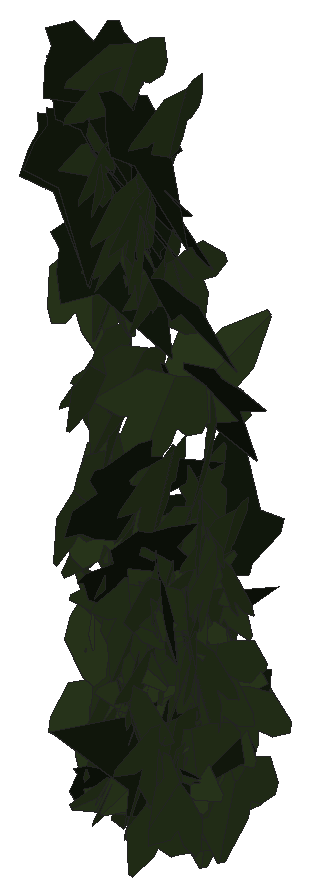
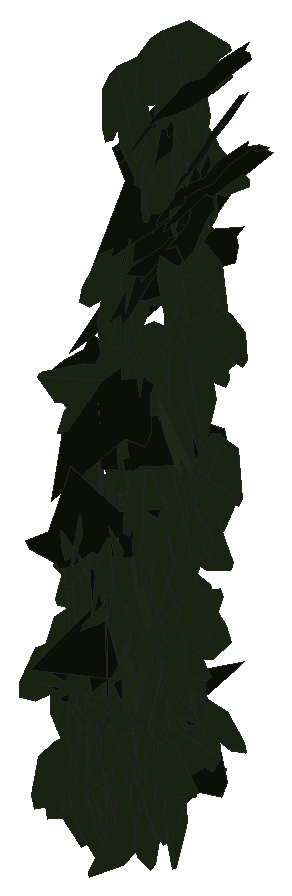
# SketchUp Ruby script. Lengths in inches.
U = 1.inch
M = Sketchup.active_model
def pt(a) = Geom::Point3d.new(a.map { |v| v * U })
def face(e, loops, mat)
  f = e.add_face(loops[0].map { |a| pt(a) })
  loops[1..].each { |l| e.add_face(l.map { |a| pt(a) }).erase! }
  f.material = f.back_material = mat if mat
  f
end
# faces: each face lists its corners as indices into pts; further lists are holes
def faces(e, pts, list, mat = nil) = list.each { |f| face(e, (f[0].is_a?(Array) ? f : [f]).map { |l| l.map { |i| pts[i] } }, mat) }
# xy, xz, yz: faces in a plane at the given z, y or x. An outline is a flat list of corners, or four numbers for a rectangle; further outlines are holes
def ring(l) = l.size == 4 ? [[l[0], l[1]], [l[2], l[1]], [l[2], l[3]], [l[0], l[3]]] : l.each_slice(2).to_a
def flat(e, list, mat, &to3) = list.each { |f| face(e, (f[0].is_a?(Array) ? f : [f]).map { |l| ring(l).map { |u, v| to3.(u, v) } }, mat) }
def xy(e, z, list, mat = nil) = flat(e, list, mat) { |x, y| [x, y, z] }
def xz(e, y, list, mat = nil) = flat(e, list, mat) { |x, z| [x, y, z] }
def yz(e, x, list, mat = nil) = flat(e, list, mat) { |y, z| [x, y, z] }
def lines(e, pts, list) = list.each { |a, b| e.add_line(pt(pts[a]), pt(pts[b])) }
# prism: a flat outline (further loops are holes) pulled along v
def prism(e, loops, v, mat = nil)
  f = face(e, loops, mat); d = Geom::Vector3d.new(v.map { |x| x * U })
  f.pushpull(f.normal.samedirection?(d) ? d.length : -d.length)
end
def box(e, o, s, mat = nil) = prism(e, [[o, [o[0] + s[0], o[1], o[2]], [o[0] + s[0], o[1] + s[1], o[2]], [o[0], o[1] + s[1], o[2]]]], [0, 0, s[2]], mat)
def at(x, y, z, deg = 0) = Geom::Transformation.translation(pt([x, y, z])) * Geom::Transformation.rotation(ORIGIN, Z_AXIS, deg.degrees)
def axes(o, x, y, z) = Geom::Transformation.new([*x, 0, *y, 0, *z, 0, *pt(o).to_a, 1])
def part(name) = M.definitions.add(name)
# library, detail: a bought-in or finely detailed component or shape, given as its bounding box
def library(name, o, s) = part(name).tap { |d| box(d.entities, o, s) }
def detail(e, o, s) = box(e.add_group.entities, o, s)
def put(e, d, t, mat = nil) = e.add_instance(d, t).tap { |i| i.material = mat if mat }
def group(e, t, mat = nil) = e.add_group.tap { |g| g.transformation = t; g.material = mat if mat }.entities
root = M.entities
M.materials.add("efeu1").color = [18, 25, 13]
M.materials.add("efeu2").color = [43, 57, 29]
c1 = part("ivyleaf_10")
p = [[0,0.5,-0.03],[-0.0625,2.02,-0.43],[-0.19,2.01,-0.46],[-0.54,1.05,-0.29],[-0.52,0.625,-0.18],[-0.83,0.76,-0.28],
  [-1.16,0.64,-0.33],[-1.15,0.33,-0.24],[-0.77,-0.39,0.02],[-0.3,-0.51,0.16],[0.04,-0.48,0.23],[-0.02,2.01,-0.4375],
  [-0.06,2.01,-0.43],[0.04,-0.49,0.23],[0.67,-0.49,0.14],[1.38,0.36,-0.2],[1.375,0.51,-0.24],[0.81,0.65,-0.19],
  [0.62,0.59,-0.15],[0.6,1.09,-0.28],[0.5,1.23,-0.31]]
faces(c1.entities,p,[[0,1,2,3,4,5,6,7,8,9,10],[11,12,0,13,14,15,16,17,18,19,20]],"efeu2")
c2 = part("ivyleaf_9")
p = [[1.54,2.16,1.25],[1.36,2.04,1.19],[-0.21,0.99,0.68],[-0.71,1.11,0.82],[-0.85,0.86,0.67],[-0.8,0.17,0.21],
  [-0.9,-0.01,0.1],[-0.67,-0.16,-0.02],[-0.08,-0.08,-0.05],[-0.03,-0.6,-0.4],[0.65,-0.88,-0.66],[0.83,-0.6,-0.49],
  [1.29,-0.42,-0.43],[1.8125,-0.07,-0.26],[1.21,0.44,0.15]]
faces(c2.entities,p,[[0,1,2,3,4,5,6,7,8,9,10,11,12,13,14]],"efeu1")
put(root,c1,axes([20.19,225.1,217.79],[0.39743,-0.18296,0.24203],[0.22039,-0.10004,-0.43752],[0.20852,0.45444,0.00113]))
put(root,c1,axes([20.46,225.47,214.79],[-0.23545,-0.43042,0.09643],[0.00497,-0.11189,-0.48729],[0.44107,-0.22851,0.05697]))
put(root,c2,axes([20.15,224.8,222.28],[0.23497,-0.44084,0.0212],[0.00899,-0.01923,-0.49955],[0.44126,0.23514,-0.00111]))
put(root,c2,axes([20.24,224.66,221.64],[0.02616,-0.49928,-0.00592],[-0.00019,0.00592,-0.49996],[0.49931,0.02617,0.00012]))
put(root,c1,axes([20.49,225.34,215.54],[-0.20462,0.40935,0.20141],[-0.12185,0.16368,-0.45647],[-0.43964,-0.23589,0.03278]))
put(root,c1,axes([20.16,224.74,220.09],[0.40688,-0.01891,0.28999],[0.2906,0.02548,-0.40608],[0.00058,0.49899,0.03173]))
put(root,c1,axes([20.45,225.24,215.66],[0.00255,-0.3876,0.31585],[0.05941,-0.31338,-0.38505],[0.49645,0.03949,0.04445]))
put(root,c1,axes([20.52,225.54,214.8],[-0.48712,-0.11246,0.00809],[-0.00902,0.00313,-0.49991],[0.11239,-0.48718,-0.00508]))
put(root,c1,axes([20.78,224.92,215.99],[-0.32902,0.02755,-0.37548],[-0.37348,0.03904,0.33013],[0.04751,0.49771,-0.00511]))
put(root,c1,axes([20.54,225.05,214.4],[0.0946,-0.46766,-0.14947],[-0.03543,0.14532,-0.4771],[0.48969,0.10086,-0.00564]))
put(root,c2,axes([20.34,224.68,221.68],[-0.01452,-0.49971,0.00885],[-0.00778,-0.00863,-0.49986],[0.49973,-0.01466,-0.00753]))
put(root,c1,axes([20.36,224.76,215.13],[0.49277,-0.02747,0.08014],[0.08002,-0.00438,-0.49354],[0.02781,0.49923,0.00008]))
put(root,c1,axes([20.51,224.86,215.05],[0.0426,-0.42233,-0.26424],[0.02584,0.26672,-0.42213],[0.49751,0.02231,0.04455]))
put(root,c1,axes([20.52,225.05,215.43],[-0.00961,-0.46549,-0.18227],[0.02388,0.18167,-0.46522],[0.49934,-0.01765,0.01874]))
put(root,c1,axes([20.49,225.57,214.2],[-0.01375,-0.2044,-0.45611],[0.09934,0.44606,-0.20289],[0.48984,-0.0962,0.02834]))
put(root,c1,axes([20.58,224.66,221.6875],[-0.2004,-0.45634,-0.03989],[0.01564,0.0367,-0.49841],[0.45782,-0.20101,-0.00044]))
put(root,c1,axes([20.52,224.8125,217.28],[-0.1788,-0.41316,-0.21755],[0.09802,0.19455,-0.45005],[0.45653,-0.20359,0.01142]))
put(root,c1,axes([20.47,224.7,220.61],[-0.46523,0.06644,-0.17071],[0.15199,-0.12007,-0.46096],[-0.10225,-0.4808,0.09152]))
put(root,c1,axes([20.56,225.32,215.68],[-0.34632,0.36037,0.01387],[-0.01897,0.001,-0.49964],[-0.36014,-0.3466,0.01298]))
put(root,c1,axes([20.6,224.61,219.31],[0.02965,-0.49785,-0.03554],[-0.00729,0.03517,-0.49871],[0.49907,0.03009,-0.00517]))
put(root,c1,axes([20.57,224.19,217.89],[0.01739,-0.35703,-0.34961],[0.07616,0.34763,-0.35121],[0.49386,-0.04104,0.06647]))
put(root,c1,axes([20.53,225.05,218.85],[0.23843,-0.39251,0.19771],[0.09728,-0.17222,-0.45921],[0.42859,0.25745,-0.00576]))
put(root,c1,axes([20.77,225.37,215.24],[-0.30241,0.29707,0.26514],[-0.22357,0.14883,-0.42175],[-0.3295,-0.37363,0.04282]))
put(root,c2,axes([20.42,224.63,222.86],[0.10015,-0.47821,-0.10621],[-0.00212,0.10798,-0.4882],[0.48986,0.09824,0.01961]))
put(root,c1,axes([20.66,224.54,221.84],[0.20046,-0.39462,-0.23257],[-0.00902,0.25041,-0.43268],[0.45797,0.17767,0.09327]))
put(root,c1,axes([20.61,225.54,214.67],[0.30361,-0.38154,0.11067],[0.06919,-0.08637,-0.4876],[0.39119,0.3114,0.00035]))
put(root,c1,axes([20.67,224.79,220.58],[0.09293,-0.44975,0.19771],[0.07221,-0.18653,-0.45825],[0.48595,0.11372,0.03029]))
put(root,c1,axes([20.89,225.07,214.92],[-0.43836,-0.18559,0.15297],[-0.12764,-0.09,-0.47498],[0.20383,-0.45548,0.03153]))
put(root,c1,axes([20.79,225.375,215.12],[-0.10944,-0.4812,0.08042],[0.0003,-0.08249,-0.49315],[0.48788,-0.10789,0.01835]))
put(root,c1,axes([20.74,224.88,216.8],[0.31348,-0.38944,-0.00831],[-0.0071,0.00496,-0.49993],[0.38946,0.31355,-0.00242]))
put(root,c2,axes([20.48,224.68,221.46],[0.47483,-0.15569,-0.0171],[-0.01874,-0.0023,-0.49964],[0.1555,0.47514,-0.00803]))
put(root,c1,axes([20.74,224.27,219.41],[-0.05005,-0.33522,-0.36759],[0.06761,0.36143,-0.33881],[0.49287,-0.08363,0.00915]))
put(root,c2,axes([20.55,224.68,220.76],[0.06467,-0.39775,-0.29599],[0.01513,0.29994,-0.39976],[0.49557,0.04275,0.05083]))
put(root,c1,axes([20.97,225.1,214.46],[0.0385,0.18611,-0.46247],[-0.37659,-0.29308,-0.14929],[-0.32665,0.35981,0.11761]))
put(root,c1,axes([20.78,224.46,221.9375],[0.11649,-0.4683,-0.13085],[-0.00118,0.13428,-0.48163],[0.48624,0.11252,0.03018]))
put(root,c1,axes([20.83,224.48,222.67],[-0.02258,-0.49943,0.00772],[-0.0009,-0.00768,-0.49994],[0.49949,-0.02259,-0.00056]))
put(root,c1,axes([20.81,225.37,215.78],[0.16447,-0.46537,-0.07989],[0.00333,0.08574,-0.49258],[0.47216,0.1615,0.0313]))
put(root,c1,axes([20.86,224.7,219.28],[-0.08703,-0.44966,0.20057],[-0.02395,-0.19957,-0.45782],[0.49178,-0.0893,0.0132]))
put(root,c1,axes([20.55,224.55,217.63],[0.25156,0.25973,0.34533],[0.22017,0.26678,-0.36104],[-0.37181,0.33371,0.01985]))
put(root,c2,axes([20.75,224.6,214.5625],[0.36265,0.33963,-0.056],[-0.04482,-0.03406,-0.49682],[-0.34129,0.36536,0.00575]))
put(root,c1,axes([20.84,225.08,217.76],[0.02903,-0.46853,-0.17216],[0.00085,0.1725,-0.4693],[0.49916,0.02696,0.01081]))
put(root,c1,axes([20.43,224.59,216.22],[0.19227,0.02749,0.46073],[0.4461,0.11702,-0.19315],[-0.11845,0.48534,0.02048]))
put(root,c1,axes([20.92,225.29,215.1875],[-0.32735,-0.3198,0.20141],[-0.06173,-0.21764,-0.44589],[0.37287,-0.3168,0.10301]))
put(root,c1,axes([20.82,225.26,215.79],[0.18501,-0.45899,0.0714],[0.01919,-0.06923,-0.49481],[0.46411,0.18583,-0.008]))
put(root,c1,axes([20.85,224.93,216.03],[0.18615,-0.42492,-0.18652],[-0.01623,0.19488,-0.46017],[0.46377,0.17738,0.05876]))
put(root,c1,axes([20.86,224.56,217.32],[0.18408,-0.46107,-0.0594],[-0.01608,0.05753,-0.49642],[0.4646,0.18467,0.00635]))
put(root,c1,axes([20.8125,225.14,216.88],[0.1828,-0.41535,0.20992],[0.10141,-0.18457,-0.45349],[0.4542,0.20838,0.01676]))
put(root,c1,axes([20.74,224.71,214.92],[0.49077,0.02428,-0.09252],[0.09107,0.02919,0.49077],[0.02923,-0.49856,0.02423]))
put(root,c1,axes([20.95,224.53,222.95],[-0.1359,-0.47419,0.08171],[-0.01698,-0.08013,-0.49324],[0.48088,-0.13684,0.00568]))
put(root,c1,axes([20.79,225.24,216.375],[-0.39917,0.26181,-0.14872],[0.11739,-0.0921,-0.47722],[-0.27728,-0.4159,0.01206]))
put(root,c1,axes([20.81,225.33,215.25],[0.49154,0.09136,0.00624],[-0.00294,0.0498,-0.49751],[-0.09152,0.48905,0.04949]))
put(root,c1,axes([20.95,224.83,214.58],[0.14383,-0.40603,-0.25388],[-0.02627,0.25799,-0.42749],[0.47815,0.13631,0.05288]))
put(root,c1,axes([20.84,225.07,215.9],[-0.01312,0.49073,-0.09495],[0.00821,-0.09476,-0.49087],[-0.49976,-0.01444,-0.00557]))
put(root,c1,axes([20.73,224.93,216.42],[0.3955,0.25632,0.16699],[0.14064,0.09004,-0.47129],[-0.27167,0.41976,-0.00087]))
put(root,c1,axes([21.02,225,215.46],[-0.19986,-0.39261,0.23645],[-0.0261,-0.24779,-0.4335],[0.45757,-0.18562,0.07856]))
put(root,c1,axes([20.98,225.22,216.17],[-0.4779,0.14368,0.0311],[-0.0299,0.00857,-0.49903],[-0.14394,-0.47883,0.0004]))
put(root,c1,axes([21.15,224.94,214.83],[0.34425,0.16796,-0.32137],[-0.30822,-0.09791,-0.38133],[-0.19103,0.46065,0.03612]))
put(root,c1,axes([21.02,224.82,215.89],[0.13846,-0.47811,0.04729],[0.00302,-0.04834,-0.49765],[0.48044,0.13809,-0.0105]))
put(root,c2,axes([21.26,224.96,214.74],[-0.09879,-0.03531,0.48887],[-0.43178,-0.22974,-0.10385],[0.23196,-0.44269,0.0149]))
put(root,c1,axes([21.02,225.2,215.09],[-0.03032,0.38567,0.31676],[-0.07904,0.30963,-0.38456],[-0.49278,-0.07339,0.0422]))
put(root,c1,axes([21.15,224.45,216.81],[-0.39963,-0.28212,0.10345],[-0.08238,-0.06268,-0.48917],[0.28898,-0.40802,0.00362]))
put(root,c1,axes([21.04,225.09,214.39],[0.00394,-0.42728,-0.25965],[0.05355,0.25853,-0.42461],[0.49711,-0.02446,0.04779]))
put(root,c1,axes([21.1,225.52,214.63],[-0.12623,-0.46988,0.11521],[-0.01296,-0.11574,-0.48625],[0.48363,-0.12575,0.01704]))
put(root,c1,axes([21.09,225.37,214.75],[-0.24971,-0.43149,0.03815],[0.01975,-0.05533,-0.49654],[0.43273,-0.24648,0.04468]))
put(root,c1,axes([21.12,225.08,216.5625],[0.45962,-0.09646,-0.1716],[-0.17036,0.02347,-0.4695],[0.09863,0.49005,-0.01129]))
put(root,c1,axes([21.06,225.45,214.68],[0.21078,-0.44951,-0.0593],[0.00947,0.06975,-0.49502],[0.4533,0.20755,0.03791]))
put(root,c1,axes([21,225.47,214.98],[0.32902,-0.37388,0.0442],[0.06316,-0.00305,-0.49598],[0.37115,0.33197,0.04522]))
put(root,c1,axes([21.1,224.63,216.79],[-0.03393,-0.46059,0.19158],[0.01502,-0.19288,-0.46106],[0.49862,-0.02553,0.02693]))
put(root,c1,axes([21.11,224.4,221.03],[0.34825,-0.29704,-0.20122],[-0.08153,0.20757,-0.44751],[0.34939,0.3445,0.09614]))
put(root,c1,axes([21.13,224.83,220.46],[0.06221,-0.41872,-0.2661],[-0.01972,0.26588,-0.42299],[0.49572,0.06312,0.01656]))
put(root,c1,axes([21.06,224.91,216.21],[0.14918,0.46996,0.08298],[-0.08147,0.11074,-0.48073],[-0.47022,0.12991,0.10961]))
put(root,c2,axes([20.9,224.58,221.58],[0.49328,0.00728,-0.08135],[-0.0814,0.00279,-0.49332],[-0.00673,0.49994,0.00393]))
put(root,c1,axes([21.02,224.5,215.52],[-0.42732,0.22128,-0.13575],[0.11399,-0.07496,-0.48103],[-0.23324,-0.44206,0.01362]))
put(root,c1,axes([21.13,224.55,221.39],[0.11539,-0.47799,-0.09062],[-0.00323,0.09238,-0.49138],[0.48649,0.11398,0.01823]))
put(root,c2,axes([20.99,224.05,218.15],[-0.02396,0.25402,-0.43],[-0.05825,0.42614,0.25498],[0.49602,0.06231,0.00917]))
put(root,c1,axes([21.05,224.95,214.7],[0.47333,0.15582,-0.04097],[-0.03868,-0.0135,-0.49832],[-0.1564,0.47491,-0.00073]))
put(root,c2,axes([20.98,225.09,216.04],[0.15719,0.22433,0.41829],[0.25812,0.32938,-0.27365],[-0.39833,0.30196,-0.01226]))
put(root,c1,axes([21.16,224.36,221.61],[-0.02477,-0.46164,-0.19045],[0.02868,0.18906,-0.46199],[0.49856,-0.03381,0.01711]))
put(root,c1,axes([21.16,225.34,216.3],[0.06775,0.41524,-0.27016],[-0.09352,-0.25706,-0.41854],[-0.48648,0.10724,0.04284]))
put(root,c1,axes([21.21,225.45,214.71],[0.02723,-0.489,-0.1007],[0.00219,0.10096,-0.4897],[0.49925,0.02623,0.00764]))
put(root,c1,axes([21.27,225.03,216.1875],[0.27125,0.29284,-0.30111],[-0.23578,-0.19048,-0.39765],[-0.3476,0.35772,0.03476]))
put(root,c1,axes([20.9,224.99,216.52],[-0.10015,0.07352,-0.48432],[0.30304,-0.37909,-0.12022],[-0.38488,-0.31762,0.03137]))
put(root,c1,axes([21.19,224.98,220.36],[-0.19524,-0.43035,-0.16334],[0.06908,0.14802,-0.47256],[0.45509,-0.2071,0.00166]))
put(root,c2,axes([20.98,224.9,220.48],[0.40999,-0.2526,-0.13455],[-0.09243,0.1056,-0.4799],[0.27087,0.41838,0.03989]))
put(root,c2,axes([21.43,225.04,216.15],[0.05058,-0.00662,-0.49739],[-0.47435,0.14991,-0.05024],[0.14979,0.47695,0.00888]))
put(root,c2,axes([21.4,224.44,217.15],[0.17032,0.00414,-0.47008],[-0.46723,0.05658,-0.16879],[0.0518,0.49677,0.02314]))
put(root,c1,axes([21.125,225.08,214.65],[0.05682,0.27911,0.41093],[0.01121,0.41279,-0.28192],[-0.49663,0.04125,0.04065]))
put(root,c1,axes([21.23,225.26,214.97],[0.14534,-0.45972,-0.13242],[0.00697,0.14042,-0.47983],[0.47836,0.13763,0.04723]))
put(root,c1,axes([21.25,225.08,216.89],[-0.42568,-0.26004,0.03436],[0.02561,-0.10639,-0.48788],[0.26104,-0.4136,0.10389]))
put(root,c1,axes([21.31,225.34,216.68],[0.46266,0.03737,-0.18588],[-0.18807,0.15252,-0.43745],[0.02401,0.4747,0.15519]))
put(root,c1,axes([21.28,225.45,214.3],[-0.30115,-0.39419,0.06263],[0.02603,-0.09769,-0.48967],[0.39829,-0.29167,0.07936]))
put(root,c2,axes([21.64,225.4,215.13],[-0.31285,0.04751,0.38713],[-0.38532,0.03925,-0.31621],[-0.06043,-0.49619,0.01205]))
put(root,c2,axes([21.17,224.07,217.39],[0.25499,0.37796,0.20524],[0.11864,0.16753,-0.45591],[-0.41341,0.28121,-0.00425]))
put(root,c1,axes([21.34,224.64,219.14],[-0.25785,-0.38367,0.19056],[-0.01542,-0.21396,-0.45164],[0.42811,-0.23879,0.09851]))
put(root,c1,axes([21.2,224.85,217.32],[0.13567,0.47467,-0.07925],[-0.0141,-0.07839,-0.49362],[-0.48103,0.13618,-0.00788]))
put(root,c2,axes([21.17,225.17,219.06],[0.46031,0.16574,-0.10319],[-0.09892,-0.02985,-0.48921],[-0.16832,0.47079,0.00531]))
put(root,c1,axes([21.19,224.6875,214.25],[-0.07797,-0.33606,-0.36192],[0.18056,0.32164,-0.33756],[0.45969,-0.18333,0.0712]))
put(root,c2,axes([21.02,224.54,222.3],[0.25583,-0.42957,0.00462],[0.00735,-0.001,-0.49995],[0.42953,0.25587,0.0058]))
put(root,c2,axes([21.36,225.38,217.05],[-0.36192,-0.1567,0.30734],[0.28509,0.11497,0.39434],[-0.19426,0.46068,0.00612]))
put(root,c1,axes([21.42,224.74,215.87],[0.25628,-0.38858,-0.18254],[-0.10011,0.15264,-0.46549],[0.41749,0.27514,0.00044]))
put(root,c1,axes([21.27,225.31,215.74],[0.00464,0.49875,-0.03496],[-0.00446,-0.03492,-0.49876],[-0.49996,0.00494,0.00413]))
put(root,c1,axes([21.3,224.9,217.48],[0.10263,-0.44462,0.20439],[0.09317,-0.18727,-0.45415],[0.4804,0.13131,0.04442]))
put(root,c1,axes([21.42,225.08,216.52],[-0.11236,-0.45583,0.17204],[-0.0354,-0.16845,-0.46944],[0.48592,-0.11767,0.00558]))
put(root,c1,axes([21.38,224.78,222.46],[0.02427,-0.49941,-0.00065],[0,0.00065,-0.5],[0.49941,0.02427,0.00003]))
put(root,c1,axes([21.35,225.05,214.87],[-0.04863,-0.44824,-0.21614],[0.05575,0.2109,-0.4499],[0.4945,-0.06786,0.02947]))
put(root,c1,axes([21.44,225.08,215.66],[-0.49196,-0.06294,0.06339],[-0.05604,-0.05888,-0.49335],[0.06957,-0.49252,0.05088]))
put(root,c1,axes([21.32,225.4,215.65],[0.42082,0.26255,-0.06309],[-0.06207,-0.01963,-0.49574],[-0.26279,0.42507,0.01608]))
put(root,c1,axes([21.41,224.61,215.24],[-0.0531,-0.49716,0.00326],[-0.00032,-0.00324,-0.49999],[0.49717,-0.05311,0.00002]))
put(root,c1,axes([21.3,225.39,215.05],[0.4998,-0.01216,-0.00691],[-0.00686,0.00202,-0.49995],[0.01219,0.49985,0.00185]))
put(root,c1,axes([21.64,224.42,214.72],[-0.37156,0.12655,0.30972],[-0.32319,-0.01607,-0.38117],[-0.08653,-0.48345,0.09374]))
put(root,c1,axes([21.43,225.3,216.94],[-0.45385,0.20072,0.06108],[-0.0503,0.03723,-0.49607],[-0.20369,-0.45643,-0.01361]))
put(root,c1,axes([21.42,224.5,218.375],[0.05456,-0.49683,-0.0137],[0.00028,0.01381,-0.49981],[0.49701,0.05454,0.00179]))
put(root,c1,axes([21.26,224.59,216.54],[-0.00339,-0.33281,0.37313],[0.09294,0.36622,0.32749],[-0.49128,0.07158,0.05938]))
put(root,c1,axes([21.52,225.11,217.76],[-0.20565,0.30037,0.34276],[-0.1961,0.28113,-0.36402],[-0.4114,-0.28415,0.00217]))
put(root,c1,axes([21.45,224.95,215.01],[-0.33304,-0.37047,-0.04293],[0.02779,0.03274,-0.49815],[0.37191,-0.33419,-0.00121]))
put(root,c1,axes([21.45,224.95,216.07],[-0.47316,0.16162,0.0019],[-0.00179,0.00063,-0.5],[-0.16162,-0.47316,-0.00002]))
put(root,c1,axes([21.32,225.21,219.04],[0.20071,0.15205,-0.43197],[0.18147,0.40662,0.22745],[0.42046,-0.24808,0.10804]))
put(root,c1,axes([21.55,225.17,215.92],[-0.29324,-0.40395,0.02895],[-0.01635,-0.02391,-0.49916],[0.40465,-0.29369,0.00082]))
put(root,c1,axes([21.54,224.84,217.86],[0.32459,-0.29148,-0.2443],[-0.09642,0.24761,-0.42355],[0.36789,0.32207,0.10453]))
put(root,c1,axes([21.55,225.48,214.41],[-0.19454,-0.45608,0.0644],[0.01389,-0.07569,-0.49404],[0.46039,-0.19043,0.04212]))
put(root,c1,axes([21.7,224.58,216.3],[-0.00507,-0.02113,-0.49953],[-0.19892,0.4584,-0.01737],[0.4587,0.19856,-0.01305]))
put(root,c1,axes([21.63,224.96,218.64],[0.22293,-0.37263,-0.24788],[-0.08706,0.23553,-0.43237],[0.439,0.23594,0.04013]))
put(root,c1,axes([21.65,224.95,217.03],[0.21234,-0.4106,-0.19059],[-0.07646,0.17496,-0.46211],[0.44617,0.22539,0.01151]))
put(root,c1,axes([21.62,225.26,217.43],[0.05997,-0.49522,0.03403],[0.00699,-0.03343,-0.49883],[0.49634,0.06031,0.00291]))
put(root,c1,axes([21.71,225.27,215.4375],[-0.44351,-0.22568,0.04867],[-0.03841,-0.03182,-0.49751],[0.22765,-0.44503,0.01089]))
put(root,c1,axes([21.74,224.73,217.34],[0.33402,-0.29624,-0.2251],[-0.16153,0.15704,-0.44637],[0.33517,0.37091,0.00921]))
